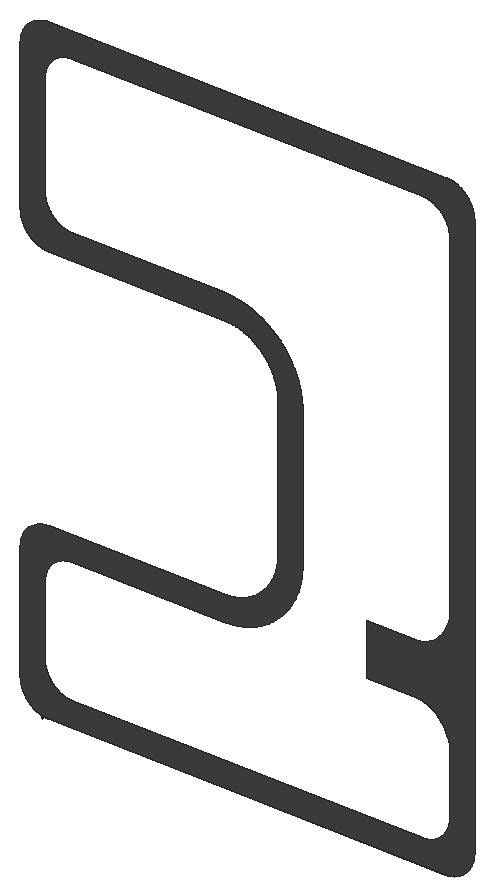
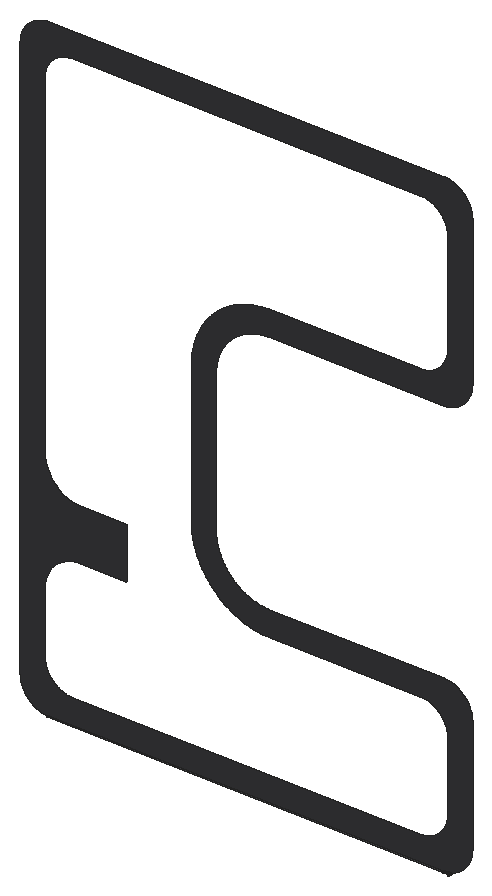
# SketchUp Ruby script. Lengths in inches.
U = 1.inch
M = Sketchup.active_model
def pt(a) = Geom::Point3d.new(a.map { |v| v * U })
def face(e, loops, mat)
  f = e.add_face(loops[0].map { |a| pt(a) })
  loops[1..].each { |l| e.add_face(l.map { |a| pt(a) }).erase! }
  f.material = f.back_material = mat if mat
  f
end
# faces: each face lists its corners as indices into pts; further lists are holes
def faces(e, pts, list, mat = nil) = list.each { |f| face(e, (f[0].is_a?(Array) ? f : [f]).map { |l| l.map { |i| pts[i] } }, mat) }
# xy, xz, yz: faces in a plane at the given z, y or x. An outline is a flat list of corners, or four numbers for a rectangle; further outlines are holes
def ring(l) = l.size == 4 ? [[l[0], l[1]], [l[2], l[1]], [l[2], l[3]], [l[0], l[3]]] : l.each_slice(2).to_a
def flat(e, list, mat, &to3) = list.each { |f| face(e, (f[0].is_a?(Array) ? f : [f]).map { |l| ring(l).map { |u, v| to3.(u, v) } }, mat) }
def xy(e, z, list, mat = nil) = flat(e, list, mat) { |x, y| [x, y, z] }
def xz(e, y, list, mat = nil) = flat(e, list, mat) { |x, z| [x, y, z] }
def yz(e, x, list, mat = nil) = flat(e, list, mat) { |y, z| [x, y, z] }
def lines(e, pts, list) = list.each { |a, b| e.add_line(pt(pts[a]), pt(pts[b])) }
# prism: a flat outline (further loops are holes) pulled along v
def prism(e, loops, v, mat = nil)
  f = face(e, loops, mat); d = Geom::Vector3d.new(v.map { |x| x * U })
  f.pushpull(f.normal.samedirection?(d) ? d.length : -d.length)
end
def box(e, o, s, mat = nil) = prism(e, [[o, [o[0] + s[0], o[1], o[2]], [o[0] + s[0], o[1] + s[1], o[2]], [o[0], o[1] + s[1], o[2]]]], [0, 0, s[2]], mat)
def at(x, y, z, deg = 0) = Geom::Transformation.translation(pt([x, y, z])) * Geom::Transformation.rotation(ORIGIN, Z_AXIS, deg.degrees)
def axes(o, x, y, z) = Geom::Transformation.new([*x, 0, *y, 0, *z, 0, *pt(o).to_a, 1])
def part(name) = M.definitions.add(name)
# library, detail: a bought-in or finely detailed component or shape, given as its bounding box
def library(name, o, s) = part(name).tap { |d| box(d.entities, o, s) }
def detail(e, o, s) = box(e.add_group.entities, o, s)
def put(e, d, t, mat = nil) = e.add_instance(d, t).tap { |i| i.material = mat if mat }
def group(e, t, mat = nil) = e.add_group.tap { |g| g.transformation = t; g.material = mat if mat }.entities
root = M.entities
M.materials.add("1432 AP 8245 TAR ROAD").color = [71, 72, 75]
M.materials.add("Outer Light").color = [251, 217, 152]
xy(root,172.79,[[278.7,95.37,278.85,96.87],[278.85,95.37,279,96.87],[279,95.37,537,96.87],[537,95.37,537.15,96.87],[537.15,95.37,537.3,96.87]],"1432 AP 8245 TAR ROAD")
xy(root,172.79,[[278.7,95.37,278.85,96.87],[278.85,95.37,279,96.87],[279,95.37,537,96.87],[537,95.37,537.15,96.87],[537.15,95.37,537.3,96.87]],"Outer Light")
xy(root,172.8,[[278.4,95.37,278.55,96.87],[537.45,95.37,537.6,96.87]],"1432 AP 8245 TAR ROAD")
xy(root,172.8,[[278.4,95.37,278.55,96.87],[537.45,95.37,537.6,96.87]],"Outer Light")
xz(root,95.37,[[[278.7,172.79,537.3,172.79,537.45,172.8,537.6,172.8,537.75,172.81,537.9,172.8125,538.04,172.82,538.64,172.86,538.79,172.875,538.9375,172.89,539.08,172.91,539.23,172.92,539.68,172.98,539.82,173,539.97,173.03,540.27,173.07,540.41,173.1,540.71,173.16,540.85,173.1875,541,173.22,541.14,173.25,541.29,173.28,541.44,173.32,541.58,173.35,541.73,173.39,542.01,173.47,542.16,173.51,542.44,173.59,542.59,173.63,542.73,173.68,542.87,173.72,543.15,173.82,543.3,173.87,543.4375,173.92,543.58,173.97,543.86,174.07,543.99,174.125,544.13,174.18,544.41,174.3,544.55,174.35,544.68,174.41,544.82,174.48,544.95,174.54,545.09,174.6,545.22,174.66,545.36,174.73,545.49,174.8,545.625,174.86,545.76,174.93,546.28,175.21,546.41,175.29,546.54,175.36,546.67,175.4375,546.8,175.51,546.93,175.59,547.05,175.67,547.31,175.83,547.43,175.91,547.56,175.99,547.68,176.08,547.8,176.16,547.93,176.25,548.05,176.33,548.41,176.6,548.53,176.6875,548.65,176.78,548.76,176.87,548.88,176.96,549,177.06,549.11,177.15,549.23,177.25,549.34,177.34,549.56,177.54,549.68,177.64,550.01,177.94,550.22,178.15,550.33,178.25,550.54,178.46,550.64,178.57,550.75,178.68,550.85,178.79,550.95,178.89,551.05,179,551.15,179.12,551.45,179.45,551.54,179.57,551.64,179.68,551.73,179.8,551.83,179.91,552.1,180.27,552.19,180.38,552.28,180.5,552.46,180.75,552.54,180.87,552.63,180.99,552.71,181.11,552.8,181.24,552.88,181.36,552.96,181.49,553.04,181.61,553.12,181.74,553.2,181.86,553.28,181.99,553.35,182.12,553.43,182.25,553.5,182.38,553.58,182.51,553.86,183.03,553.93,183.17,554,183.3,554.0625,183.43,554.13,183.57,554.19,183.7,554.25,183.84,554.32,183.97,554.38,184.11,554.4375,184.25,554.5,184.38,554.55,184.52,554.67,184.8,554.72,184.9375,554.77,185.08,554.83,185.22,554.875,185.36,554.93,185.5,554.98,185.64,555.02,185.78,555.07,185.92,555.12,186.0625,555.16,186.21,555.2,186.35,555.25,186.49,555.29,186.63,555.33,186.78,555.37,186.92,555.4,187.07,555.44,187.21,555.48,187.36,555.51,187.5,555.54,187.65,555.57,187.79,555.61,187.9375,555.63,188.09,555.66,188.23,555.72,188.53,555.74,188.67,555.77,188.82,555.79,188.97,555.81,189.11,555.89,189.71,555.9,189.86,555.92,190,555.99,191.05,555.99,191.34,556,191.49,556,561.09,555.99,561.24,555.99,561.54,555.98,561.6875,555.97,561.84,555.96,561.99,555.95,562.13,555.92,562.58,555.9,562.73,555.89,562.88,555.87,563.03,555.85,563.17,555.79,563.62,555.77,563.76,555.74,563.91,555.72,564.06,555.69,564.21,555.66,564.35,555.63,564.5,555.61,564.65,555.57,564.79,555.54,564.9375,555.51,565.08,555.48,565.23,555.44,565.37,555.4,565.52,555.37,565.66,555.33,565.81,555.25,566.09,555.2,566.24,555.12,566.52,555.07,566.66,555.02,566.81,554.98,566.95,554.93,567.09,554.875,567.23,554.83,567.37,554.77,567.51,554.67,567.79,554.61,567.92,554.55,568.0625,554.5,568.2,554.4375,568.34,554.38,568.47,554.32,568.61,554.25,568.75,554.19,568.88,554.13,569.02,554.0625,569.15,554,569.28,553.93,569.42,553.79,569.68,553.72,569.8125,553.65,569.95,553.58,570.08,553.5,570.21,553.43,570.34,553.35,570.46,553.28,570.59,553.12,570.85,553.04,570.97,552.96,571.1,552.88,571.22,552.8,571.35,552.71,571.47,552.63,571.59,552.54,571.72,552.46,571.84,552.1,572.32,552.01,572.4375,551.92,572.55,551.83,572.67,551.73,572.79,551.64,572.9,551.54,573.02,551.45,573.13,551.35,573.24,551.25,573.36,551.05,573.58,550.95,573.6875,550.85,573.8,550.75,573.91,550.64,574.01,550.44,574.23,550.33,574.33,550.22,574.4375,550.11,574.54,550.01,574.64,549.9,574.74,549.79,574.85,549.68,574.95,549.56,575.04,549.23,575.34,549.11,575.43,549,575.53,548.76,575.71,548.65,575.8,548.53,575.9,548.29,576.08,548.17,576.16,547.93,576.34,547.8,576.42,547.68,576.51,547.56,576.59,547.43,576.67,547.31,576.75,547.05,576.91,546.93,576.99,546.67,577.15,546.54,577.22,546.41,577.3,545.76,577.65,545.49,577.79,545.36,577.85,545.22,577.92,545.09,577.98,544.95,578.05,544.82,578.11,544.68,578.17,544.55,578.23,544.27,578.35,544.13,578.4,543.99,578.46,543.86,578.51,543.72,578.57,543.58,578.62,543.4375,578.67,543.3,578.72,543.15,578.77,543.01,578.82,542.87,578.86,542.73,578.91,542.59,578.95,542.44,579,542.16,579.08,542.01,579.12,541.73,579.2,541.58,579.23,541.44,579.27,541.14,579.33,541,579.37,540.85,579.4,540.71,579.43,540.56,579.46,540.41,579.48,540.27,579.51,540.12,579.53,539.97,579.56,539.82,579.58,539.68,579.6,539.08,579.68,538.9375,579.69,538.79,579.71,538.04,579.76,537.9,579.77,537.75,579.78,537.6,579.78,537.45,579.79,278.55,579.79,278.4,579.78,278.25,579.78,278.1,579.77,277.96,579.76,277.21,579.71,277.0625,579.69,276.92,579.68,276.32,579.6,276.18,579.58,276.03,579.56,275.88,579.53,275.73,579.51,275.59,579.48,275.44,579.46,275.29,579.43,275.15,579.4,275,579.37,274.86,579.33,274.56,579.27,274.42,579.23,274.27,579.2,273.99,579.12,273.84,579.08,273.56,579,273.41,578.95,273.27,578.91,273.13,578.86,272.99,578.82,272.85,578.77,272.7,578.72,272.5625,578.67,272.42,578.62,272.28,578.57,272.14,578.51,272.01,578.46,271.87,578.4,271.73,578.35,271.45,578.23,271.32,578.17,271.18,578.11,271.05,578.05,270.91,577.98,270.78,577.92,270.64,577.85,270.51,577.79,270.24,577.65,269.59,577.3,269.46,577.22,269.33,577.15,269.07,576.99,268.95,576.91,268.69,576.75,268.57,576.67,268.44,576.59,268.32,576.51,268.2,576.42,268.07,576.34,267.83,576.16,267.71,576.08,267.47,575.9,267.35,575.8,267.24,575.71,267,575.53,266.89,575.43,266.77,575.34,266.44,575.04,266.32,574.95,266.21,574.85,266.1,574.74,265.99,574.64,265.89,574.54,265.78,574.4375,265.67,574.33,265.56,574.23,265.36,574.01,265.25,573.91,265.15,573.8,265.05,573.6875,264.95,573.58,264.75,573.36,264.65,573.24,264.55,573.13,264.46,573.02,264.36,572.9,264.27,572.79,264.17,572.67,264.08,572.55,263.99,572.4375,263.9,572.32,263.54,571.84,263.46,571.72,263.37,571.59,263.29,571.47,263.2,571.35,263.12,571.22,263.04,571.1,262.96,570.97,262.88,570.85,262.72,570.59,262.65,570.46,262.57,570.34,262.5,570.21,262.42,570.08,262.35,569.95,262.28,569.8125,262.21,569.68,262.07,569.42,262,569.28,261.9375,569.15,261.87,569.02,261.81,568.88,261.75,568.75,261.68,568.61,261.62,568.47,261.5625,568.34,261.5,568.2,261.45,568.0625,261.39,567.92,261.33,567.79,261.23,567.51,261.17,567.37,261.125,567.23,261.07,567.09,261.02,566.95,260.98,566.81,260.93,566.66,260.88,566.52,260.8,566.24,260.75,566.09,260.67,565.81,260.63,565.66,260.6,565.52,260.56,565.37,260.52,565.23,260.49,565.08,260.46,564.9375,260.43,564.79,260.39,564.65,260.37,564.5,260.34,564.35,260.31,564.21,260.28,564.06,260.26,563.91,260.23,563.76,260.21,563.62,260.15,563.17,260.13,563.03,260.11,562.88,260.1,562.73,260.08,562.58,260.05,562.13,260.04,561.99,260.03,561.84,260.02,561.6875,260.01,561.54,260.01,561.24,260,561.09,260,464.49,260.01,464.34,260.01,464.05,260.08,463,260.1,462.86,260.11,462.71,260.19,462.11,260.21,461.97,260.23,461.82,260.26,461.67,260.28,461.53,260.34,461.23,260.37,461.09,260.39,460.9375,260.43,460.79,260.46,460.65,260.49,460.5,260.52,460.36,260.56,460.21,260.6,460.07,260.63,459.92,260.67,459.78,260.71,459.63,260.75,459.49,260.8,459.35,260.84,459.21,260.88,459.0625,260.93,458.92,260.98,458.78,261.02,458.64,261.07,458.5,261.125,458.36,261.17,458.22,261.23,458.08,261.28,457.9375,261.33,457.8,261.45,457.52,261.5,457.38,261.5625,457.25,261.62,457.11,261.68,456.97,261.75,456.84,261.81,456.7,261.87,456.57,261.9375,456.43,262,456.3,262.07,456.17,262.14,456.03,262.42,455.51,262.5,455.38,262.57,455.25,262.65,455.12,262.72,454.99,262.8,454.86,262.88,454.74,262.96,454.61,263.04,454.49,263.12,454.36,263.2,454.24,263.29,454.11,263.37,453.99,263.46,453.87,263.54,453.75,263.72,453.5,263.81,453.38,263.9,453.27,264.17,452.91,264.27,452.8,264.36,452.68,264.46,452.57,264.55,452.45,264.85,452.12,264.95,452,265.05,451.89,265.15,451.79,265.25,451.68,265.36,451.57,265.46,451.46,265.67,451.25,265.78,451.15,265.99,450.94,266.32,450.64,266.44,450.54,266.66,450.34,266.77,450.25,266.89,450.15,267,450.06,267.12,449.96,267.24,449.87,267.35,449.78,267.47,449.6875,267.59,449.6,267.95,449.33,268.07,449.25,268.2,449.16,268.32,449.08,268.44,448.99,268.57,448.91,268.69,448.83,268.95,448.67,269.07,448.59,269.2,448.51,269.33,448.4375,269.46,448.36,269.59,448.29,269.72,448.21,270.24,447.93,270.375,447.86,270.51,447.8,270.64,447.73,270.78,447.66,270.91,447.6,271.05,447.54,271.18,447.48,271.32,447.41,271.45,447.35,271.59,447.3,271.87,447.18,272.01,447.125,272.14,447.07,272.42,446.97,272.5625,446.92,272.7,446.87,272.85,446.82,273.13,446.72,273.27,446.68,273.41,446.63,273.56,446.59,273.84,446.51,273.99,446.47,274.27,446.39,274.42,446.35,274.56,446.32,274.71,446.28,274.86,446.25,275,446.22,275.15,446.1875,275.29,446.16,275.59,446.1,275.73,446.07,276.03,446.03,276.18,446,276.32,445.98,276.77,445.92,276.92,445.91,277.0625,445.89,277.21,445.875,277.36,445.86,277.96,445.82,278.1,445.8125,278.25,445.81,278.4,445.8,278.55,445.8,278.7,445.79,393.46,445.79,393.92,445.78,394.375,445.77,394.83,445.74,395.29,445.72,395.75,445.68,396.2,445.65,396.66,445.6,397.11,445.55,397.57,445.49,398.02,445.43,398.48,445.36,398.93,445.29,399.38,445.21,400.28,445.03,400.72,444.93,401.17,444.82,401.62,444.72,402.5,444.48,403.38,444.22,403.82,444.08,405.11,443.63,405.54,443.47,405.97,443.3,406.39,443.13,406.82,442.95,407.24,442.77,407.65,442.58,408.07,442.38,408.89,441.98,409.3,441.77,410.1,441.33,410.9,440.87,411.68,440.39,412.0625,440.15,412.44,439.89,412.82,439.64,413.2,439.375,413.57,439.11,413.94,438.84,414.31,438.56,414.67,438.28,415.03,437.99,415.73,437.41,416.08,437.11,416.76,436.49,417.09,436.18,417.75,435.54,418.39,434.88,418.7,434.55,419.01,434.21,419.3125,433.87,419.61,433.52,419.91,433.17,420.2,432.82,420.49,432.46,420.77,432.1,421.04,431.73,421.32,431.36,421.84,430.62,422.1,430.24,422.35,429.85,422.6,429.47,422.84,429.08,423.08,428.6875,423.3125,428.29,423.54,427.89,423.76,427.49,423.97,427.09,424.19,426.68,424.79,425.45,424.97,425.03,425.16,424.61,425.34,424.1875,425.51,423.76,425.68,423.33,425.84,422.91,425.99,422.48,426.14,422.04,426.29,421.61,426.43,421.17,426.56,420.73,426.6875,420.29,426.81,419.85,426.92,419.41,427.03,418.96,427.14,418.52,427.24,418.07,427.33,417.62,427.57,416.27,427.64,415.8125,427.7,415.36,427.76,414.91,427.81,414.45,427.85,413.99,427.89,413.54,427.93,413.08,427.97,412.17,427.99,411.71,428,411.25,428,320.33,427.99,319.875,427.97,319.42,427.93,318.5,427.89,318.05,427.81,317.13,427.76,316.68,427.7,316.22,427.64,315.77,427.57,315.32,427.49,314.86,427.33,313.96,427.24,313.52,427.14,313.07,427.03,312.62,426.92,312.18,426.81,311.73,426.6875,311.29,426.56,310.85,426.43,310.41,426.29,309.98,426.14,309.54,425.84,308.68,425.68,308.25,425.51,307.82,425.34,307.4,425.16,306.98,424.97,306.56,424.79,306.14,424.59,305.72,424.39,305.3125,424.19,304.9,423.97,304.5,423.76,304.09,423.54,303.69,423.3125,303.29,423.08,302.9,422.84,302.5,422.6,302.12,422.35,301.73,422.1,301.35,421.58,300.59,421.32,300.22,421.04,299.85,420.77,299.49,420.49,299.125,420.2,298.77,419.91,298.41,419.61,298.0625,419.3125,297.71,419.01,297.37,418.7,297.03,418.39,296.7,417.75,296.04,417.09,295.4,416.76,295.09,416.42,294.78,416.08,294.48,415.38,293.88,415.03,293.59,414.67,293.31,414.31,293.02,413.2,292.21,412.44,291.69,412.0625,291.4375,411.68,291.19,410.9,290.71,410.1,290.25,409.7,290.03,409.3,289.82,408.48,289.4,408.07,289.2,407.65,289.01,407.24,288.82,406.82,288.63,406.39,288.46,405.97,288.28,404.68,287.8,404.25,287.65,403.82,287.51,402.94,287.23,402.5,287.11,402.06,286.98,401.62,286.87,401.17,286.76,400.72,286.66,400.28,286.56,399.83,286.46,398.48,286.22,398.02,286.15,397.57,286.09,397.11,286.03,396.66,285.98,396.2,285.9375,395.75,285.9,394.83,285.84,393.92,285.8,393.46,285.8,393,285.79,279,285.79,276.52,285.63,274.08,285.14,271.73,284.35,269.5,283.25,267.43,281.87,265.56,280.23,263.93,278.36,262.55,276.29,261.45,274.0625,260.65,271.71,260.16,269.27,260,266.79,260,191.49,260.01,191.34,260.01,191.05,260.08,190,260.1,189.86,260.11,189.71,260.19,189.11,260.21,188.97,260.23,188.82,260.26,188.67,260.28,188.53,260.34,188.23,260.37,188.09,260.39,187.9375,260.43,187.79,260.46,187.65,260.49,187.5,260.52,187.36,260.56,187.21,260.6,187.07,260.63,186.92,260.67,186.78,260.71,186.63,260.75,186.49,260.8,186.35,260.84,186.21,260.88,186.0625,260.93,185.92,260.98,185.78,261.02,185.64,261.07,185.5,261.125,185.36,261.17,185.22,261.23,185.08,261.28,184.9375,261.33,184.8,261.45,184.52,261.5,184.38,261.5625,184.25,261.62,184.11,261.68,183.97,261.75,183.84,261.81,183.7,261.87,183.57,261.9375,183.43,262,183.3,262.07,183.17,262.14,183.03,262.42,182.51,262.5,182.38,262.57,182.25,262.65,182.12,262.72,181.99,262.8,181.86,262.88,181.74,262.96,181.61,263.04,181.49,263.12,181.36,263.2,181.24,263.29,181.11,263.37,180.99,263.46,180.87,263.54,180.75,263.72,180.5,263.81,180.38,263.9,180.27,264.17,179.91,264.27,179.8,264.36,179.68,264.46,179.57,264.55,179.45,264.85,179.12,264.95,179,265.05,178.89,265.15,178.79,265.25,178.68,265.36,178.57,265.46,178.46,265.67,178.25,265.78,178.15,265.99,177.94,266.32,177.64,266.44,177.54,266.66,177.34,266.77,177.25,266.89,177.15,267,177.06,267.12,176.96,267.24,176.87,267.35,176.78,267.47,176.6875,267.59,176.6,267.95,176.33,268.07,176.25,268.2,176.16,268.32,176.08,268.44,175.99,268.57,175.91,268.69,175.83,268.95,175.67,269.07,175.59,269.2,175.51,269.33,175.4375,269.46,175.36,269.59,175.29,269.72,175.21,270.24,174.93,270.375,174.86,270.51,174.8,270.64,174.73,270.78,174.66,270.91,174.6,271.05,174.54,271.18,174.48,271.32,174.41,271.45,174.35,271.59,174.3,271.87,174.18,272.01,174.125,272.14,174.07,272.42,173.97,272.5625,173.92,272.7,173.87,272.85,173.82,273.13,173.72,273.27,173.68,273.41,173.63,273.56,173.59,273.84,173.51,273.99,173.47,274.27,173.39,274.42,173.35,274.56,173.32,274.71,173.28,274.86,173.25,275,173.22,275.15,173.1875,275.29,173.16,275.59,173.1,275.73,173.07,276.03,173.03,276.18,173,276.32,172.98,276.77,172.92,276.92,172.91,277.0625,172.89,277.21,172.875,277.36,172.86,277.96,172.82,278.1,172.8125,278.25,172.81,278.4,172.8,278.55,172.8],[293.76,188.79,293.53,188.8,293.29,188.81,293.06,188.82,292.82,188.83,292.59,188.85,292.35,188.87,292.12,188.89,291.88,188.92,291.42,188.98,291.18,189.01,290.72,189.09,289.8,189.29,289.11,189.47,288.89,189.53,288.66,189.6,288.4375,189.67,288.21,189.75,287.99,189.82,287.77,189.9,287.55,189.99,287.33,190.07,286.89,190.25,286.68,190.35,286.46,190.45,285.83,190.75,285.41,190.97,285.2,191.09,285,191.2,284.6,191.44,284.39,191.57,284.2,191.7,283.8,191.96,283.61,192.09,283.04,192.51,282.86,192.66,282.67,192.8,282.31,193.1,282.13,193.26,281.96,193.42,281.78,193.57,281.61,193.74,281.44,193.9,281.27,194.0625,281.11,194.23,280.94,194.4,280.78,194.57,280.625,194.75,280.47,194.92,280.3125,195.1,280.16,195.28,280.01,195.46,279.86,195.65,279.72,195.83,279.58,196.02,279.4375,196.21,279.3,196.4,279.17,196.6,279.03,196.79,278.9,196.99,278.78,197.1875,278.65,197.39,278.41,197.79,278.3,198,278.18,198.2,277.96,198.62,277.86,198.83,277.75,199.04,277.65,199.26,277.56,199.47,277.46,199.6875,277.37,199.9,277.28,200.12,277.2,200.34,277.11,200.5625,277.03,200.78,276.96,201.01,276.88,201.23,276.81,201.45,276.74,201.68,276.68,201.91,276.61,202.13,276.55,202.36,276.5,202.59,276.44,202.82,276.39,203.05,276.35,203.28,276.3,203.51,276.26,203.74,276.22,203.98,276.1875,204.21,276.15,204.44,276.125,204.68,276.1,204.91,276.08,205.15,276.04,205.61,276.02,205.85,276.01,206.09,276.01,206.32,276,206.56,276,252.19,276.01,252.4,276.04,253,276.06,253.2,276.07,253.4,276.11,253.8,276.14,254,276.16,254.2,276.25,254.8,276.29,255,276.32,255.2,276.36,255.39,276.41,255.59,276.45,255.79,276.49,255.98,276.54,256.18,276.59,256.375,276.65,256.57,276.7,256.76,276.76,256.96,276.82,257.15,276.875,257.34,277,257.72,277.21,258.29,277.29,258.48,277.36,258.66,277.44,258.85,277.52,259.03,277.6,259.22,277.6875,259.4,277.77,259.58,278.04,260.12,278.14,260.3,278.23,260.48,278.33,260.65,278.43,260.83,278.53,261,278.64,261.17,278.74,261.35,278.85,261.52,278.96,261.68,279.07,261.85,279.1875,262.02,279.3,262.18,279.42,262.35,279.78,262.83,279.91,262.99,280.03,263.15,280.16,263.3,280.29,263.46,280.55,263.76,280.6875,263.91,280.83,264.06,280.96,264.2,281.1,264.35,281.24,264.49,281.39,264.63,281.53,264.77,281.83,265.05,282,265.16,282.16,265.3125,282.33,265.46,282.49,265.61,282.67,265.76,282.84,265.9,283.01,266.03,283.19,266.17,283.37,266.3,283.56,266.43,283.74,266.55,284.12,266.79,284.27,266.9375,284.45,267.05,284.81,267.27,285.17,267.48,285.36,267.58,285.54,267.68,285.73,267.78,285.91,267.87,286.1,267.97,286.48,268.15,286.67,268.23,286.86,268.32,287.06,268.4,287.44,268.56,287.84,268.7,288.03,268.77,288.43,268.91,289.23,269.15,289.4375,269.2,289.64,269.26,289.84,269.31,290.05,269.35,290.25,269.4,290.46,269.44,290.66,269.48,290.87,269.52,291.08,269.55,291.28,269.59,291.49,269.62,291.7,269.64,291.91,269.67,292.12,269.69,292.32,269.71,292.74,269.75,293.58,269.79,393,269.79,394.34,269.81,395,269.83,395.67,269.86,396.34,269.9,397,269.95,397.67,270.01,398.33,270.07,398.99,270.15,399.66,270.23,400.32,270.32,400.98,270.42,401.64,270.53,402.29,270.65,402.95,270.77,403.6,270.91,404.26,271.05,404.91,271.2,405.55,271.36,406.2,271.53,407.48,271.89,408.125,272.09,408.76,272.29,409.39,272.5,410.65,272.94,411.28,273.18,411.9,273.42,412.52,273.67,413.13,273.93,413.74,274.2,414.96,274.76,415.56,275.05,416.15,275.35,416.75,275.66,417.34,275.97,417.92,276.29,419.08,276.96,419.65,277.31,420.21,277.66,420.78,278.02,421.33,278.39,421.89,278.76,422.43,279.14,422.98,279.53,423.51,279.93,424.05,280.33,424.57,280.74,425.1,281.16,425.61,281.58,426.12,282.01,426.625,282.45,427.125,282.89,427.62,283.34,428.11,283.8,428.59,284.26,429.0625,284.73,429.53,285.2,429.99,285.6875,430.45,286.17,430.9,286.67,431.78,287.67,432.21,288.18,433.05,289.22,433.46,289.75,433.86,290.28,434.26,290.82,434.65,291.36,435.03,291.91,435.4,292.46,435.77,293.02,436.13,293.58,436.48,294.14,436.83,294.72,437.17,295.29,437.5,295.87,437.82,296.46,438.44,297.64,438.74,298.24,439.32,299.44,439.86,300.66,440.12,301.28,440.37,301.89,440.61,302.52,440.85,303.14,441.29,304.4,441.5,305.03,441.71,305.67,442.09,306.95,442.26,307.59,442.43,308.24,442.59,308.89,442.74,309.54,442.89,310.1875,443.02,310.84,443.15,311.5,443.26,312.16,443.37,312.8125,443.47,313.47,443.5625,314.14,443.65,314.8,443.72,315.46,443.79,316.125,443.84,316.79,443.89,317.46,443.93,318.12,443.96,318.79,443.98,319.46,444,320.125,444,411.46,443.98,412.13,443.96,412.79,443.93,413.46,443.89,414.13,443.84,414.79,443.79,415.46,443.65,416.79,443.5625,417.45,443.47,418.11,443.37,418.77,443.15,420.09,443.02,420.74,442.89,421.4,442.59,422.7,442.43,423.35,442.26,423.99,442.09,424.64,441.71,425.92,441.5,426.55,441.29,427.19,441.07,427.82,440.85,428.44,440.61,429.07,440.37,429.69,440.12,430.31,439.86,430.92,439.59,431.54,439.32,432.14,439.03,432.75,438.74,433.35,438.44,433.95,437.82,435.13,437.5,435.71,437.17,436.29,436.83,436.87,436.48,437.4375,436.13,438.01,435.77,438.57,435.03,439.68,434.65,440.23,434.26,440.77,433.86,441.31,433.46,441.84,433.05,442.37,432.63,442.89,432.21,443.4,431.78,443.91,431.34,444.42,430.9,444.92,430.45,445.41,429.99,445.9,429.53,446.38,429.0625,446.85,428.59,447.32,428.11,447.79,427.62,448.24,427.125,448.69,426.625,449.14,426.12,449.57,425.1,450.43,424.57,450.84,424.05,451.25,423.51,451.66,422.98,452.05,422.43,452.44,421.89,452.82,421.33,453.2,420.78,453.5625,420.21,453.92,419.65,454.28,419.08,454.62,418.5,454.96,417.92,455.29,417.34,455.61,416.75,455.93,416.15,456.23,415.56,456.53,414.96,456.82,414.35,457.11,413.13,457.65,412.52,457.91,411.9,458.16,411.28,458.4,410.65,458.64,410.02,458.87,409.39,459.09,408.76,459.3,408.125,459.5,407.48,459.69,406.84,459.88,406.2,460.05,405.55,460.22,404.91,460.38,404.26,460.53,403.6,460.68,402.95,460.8125,402.29,460.9375,401.64,461.06,399.66,461.36,398.99,461.4375,398.33,461.51,397.67,461.58,397,461.63,396.34,461.68,395.67,461.72,395,461.75,394.34,461.77,393.67,461.79,293.76,461.79,293.53,461.8,293.29,461.81,293.06,461.82,292.82,461.83,292.59,461.85,292.35,461.87,292.12,461.89,291.88,461.92,291.42,461.98,291.18,462.01,290.72,462.09,289.8,462.29,289.11,462.47,288.89,462.53,288.66,462.6,288.4375,462.67,288.21,462.75,287.99,462.82,287.77,462.9,287.55,462.99,287.33,463.07,286.89,463.25,286.68,463.35,286.46,463.45,285.83,463.75,285.41,463.97,285.2,464.09,285,464.2,284.6,464.44,284.39,464.57,284.2,464.7,283.8,464.96,283.61,465.09,283.04,465.51,282.86,465.66,282.67,465.8,282.31,466.1,282.13,466.26,281.96,466.42,281.78,466.57,281.61,466.74,281.44,466.9,281.27,467.0625,281.11,467.23,280.94,467.4,280.78,467.57,280.625,467.75,280.47,467.92,280.3125,468.1,280.16,468.28,280.01,468.46,279.86,468.65,279.72,468.83,279.58,469.02,279.4375,469.21,279.3,469.4,279.17,469.6,279.03,469.79,278.9,469.99,278.78,470.1875,278.65,470.39,278.41,470.79,278.3,471,278.18,471.2,277.96,471.62,277.86,471.83,277.75,472.04,277.65,472.26,277.56,472.47,277.46,472.6875,277.37,472.9,277.28,473.12,277.2,473.34,277.11,473.5625,277.03,473.78,276.96,474.01,276.88,474.23,276.81,474.45,276.74,474.68,276.68,474.91,276.61,475.13,276.55,475.36,276.5,475.59,276.44,475.82,276.39,476.05,276.35,476.28,276.3,476.51,276.26,476.74,276.22,476.98,276.1875,477.21,276.15,477.44,276.125,477.68,276.1,477.91,276.08,478.15,276.04,478.61,276.02,478.85,276.01,479.09,276.01,479.32,276,479.56,276,546.03,276.01,546.26,276.01,546.5,276.02,546.73,276.04,546.97,276.06,547.2,276.08,547.4375,276.1,547.67,276.125,547.91,276.15,548.14,276.1875,548.375,276.22,548.61,276.3,549.07,276.35,549.3,276.39,549.53,276.44,549.76,276.5,549.99,276.55,550.22,276.61,550.45,276.68,550.68,276.74,550.9,276.81,551.13,276.88,551.35,276.96,551.58,277.03,551.8,277.11,552.02,277.2,552.24,277.28,552.46,277.46,552.9,277.56,553.11,277.65,553.33,277.75,553.54,277.86,553.75,277.96,553.96,278.18,554.38,278.3,554.59,278.41,554.79,278.53,555,278.65,555.2,278.78,555.4,278.9,555.6,279.03,555.79,279.17,555.99,279.3,556.18,279.4375,556.37,279.58,556.5625,279.86,556.9375,280.01,557.12,280.16,557.3,280.3125,557.48,280.47,557.66,280.625,557.84,280.78,558.01,280.94,558.18,281.11,558.35,281.27,558.52,281.44,558.69,281.78,559.01,281.96,559.17,282.13,559.33,282.67,559.78,282.86,559.93,283.04,560.07,283.61,560.49,283.8,560.625,284,560.76,284.2,560.89,284.39,561.02,284.6,561.14,285.2,561.5,285.83,561.83,286.04,561.9375,286.25,562.04,286.46,562.14,286.68,562.24,286.89,562.33,287.55,562.6,288.21,562.84,288.4375,562.91,288.66,562.98,288.89,563.05,289.11,563.12,289.57,563.24,289.8,563.29,290.03,563.35,290.49,563.45,291.18,563.57,291.42,563.61,291.88,563.67,292.12,563.69,292.35,563.72,292.59,563.74,292.82,563.75,293.06,563.77,293.29,563.78,293.53,563.79,522.4,563.79,522.61,563.78,523.41,563.74,523.81,563.7,524.02,563.68,524.22,563.66,525.02,563.54,525.21,563.5,525.41,563.47,525.61,563.43,525.81,563.38,526.01,563.34,526.2,563.29,526.4,563.25,526.59,563.2,526.79,563.14,526.98,563.09,527.18,563.03,527.37,562.97,527.5625,562.91,527.75,562.85,527.95,562.78,528.14,562.71,528.32,562.64,528.7,562.5,528.89,562.42,529.07,562.34,529.26,562.26,529.44,562.18,529.63,562.1,530.35,561.74,530.53,561.64,530.71,561.55,530.88,561.45,531.06,561.35,531.23,561.24,531.4,561.14,531.58,561.03,531.75,560.92,531.92,560.8125,532.08,560.7,532.25,560.59,532.42,560.47,532.9,560.11,533.0625,559.99,533.22,559.87,533.54,559.61,533.84,559.35,533.99,559.21,534.14,559.08,534.29,558.94,534.4375,558.8,534.58,558.66,534.73,558.52,535.01,558.23,535.15,558.08,535.29,557.9375,535.42,557.79,535.56,557.63,535.6875,557.48,535.82,557.33,535.95,557.17,536.07,557.01,536.2,556.86,536.32,556.7,536.44,556.53,536.5625,556.37,536.68,556.21,536.8,556.04,537.02,555.71,537.35,555.2,537.45,555.02,537.55,554.85,537.66,554.68,537.75,554.5,537.95,554.14,538.22,553.6,538.3,553.42,538.39,553.24,538.47,553.05,538.55,552.87,538.71,552.49,538.78,552.31,539.06,551.55,539.12,551.35,539.3,550.78,539.35,550.58,539.4,550.39,539.5,549.99,539.55,549.8,539.67,549.2,539.71,549.01,539.75,548.81,539.84,548.21,539.86,548.01,539.89,547.81,539.93,547.41,539.94,547.2,539.96,547,540,546.2,540,326.79,539.79,323.66,539.18,320.58,538.17,317.61,536.78,314.79,535.04,312.18,532.97,309.82,530.61,307.75,528,306.01,525.18,304.62,522.21,303.61,519.13,303,516,302.79,486,302.79,486,269.79,516,269.79,519.13,269.59,522.21,268.97,525.18,267.97,528,266.58,530.61,264.83,532.97,262.76,535.04,260.4,536.78,257.79,538.17,254.98,539.18,252,539.79,248.92,540,245.79,540,206.39,539.99,206.1875,539.98,205.98,539.96,205.58,539.94,205.38,539.93,205.18,539.89,204.78,539.86,204.58,539.84,204.375,539.81,204.18,539.75,203.78,539.59,202.98,539.55,202.79,539.45,202.39,539.4,202.2,539.35,202,539.3,201.81,539.24,201.62,539.18,201.42,539.06,201.04,538.71,200.09,538.63,199.9,538.55,199.72,538.47,199.53,538.39,199.35,538.3,199.16,538.22,198.98,537.95,198.44,537.85,198.26,537.75,198.09,537.66,197.91,537.55,197.73,537.35,197.39,537.13,197.05,537.02,196.875,536.91,196.71,536.8,196.54,536.68,196.375,536.5625,196.21,536.44,196.05,536.2,195.73,536.07,195.57,535.95,195.41,535.82,195.26,535.6875,195.1,535.56,194.95,535.42,194.8,535.29,194.65,535.01,194.35,534.87,194.21,534.73,194.0625,534.58,193.92,534.4375,193.78,534.29,193.64,534.14,193.51,533.99,193.37,533.84,193.24,533.69,193.1,533.54,192.97,533.38,192.85,533.22,192.72,533.0625,192.59,532.9,192.47,532.42,192.11,532.25,192,532.08,191.88,531.92,191.77,531.58,191.55,531.4,191.44,531.06,191.24,530.88,191.14,530.71,191.04,530.53,190.94,530.35,190.85,530.17,190.75,529.81,190.57,529.63,190.49,529.44,190.4,529.26,190.32,529.07,190.24,528.89,190.16,528.7,190.09,528.51,190.01,528.32,189.94,528.14,189.87,527.95,189.8,527.75,189.74,527.5625,189.67,527.37,189.61,527.18,189.55,526.98,189.5,526.79,189.44,526.59,189.39,526.4,189.34,526.2,189.29,526.01,189.24,525.21,189.08,525.02,189.05,524.82,189.01,524.42,188.95,524.02,188.91,523.81,188.88,523.61,188.86,523.41,188.85,523.21,188.83,522.61,188.8,522.4,188.8,522.2,188.79]]],"1432 AP 8245 TAR ROAD")
p = [[274.21,95.37,171.86],[274.37,95.37,171.82],[274.37,96.87,171.82],[274.21,96.87,171.86],[274.21,96.87,171.86],[274.37,96.87,171.82],
  [274.37,95.37,171.82],[274.21,95.37,171.86],[274.53,95.37,171.79],[274.53,96.87,171.79],[274.53,96.87,171.79],[274.53,95.37,171.79],
  [274.69,95.37,171.75],[274.69,96.87,171.75],[274.69,96.87,171.75],[274.69,95.37,171.75],[273.75,95.37,171.98],[273.9,95.37,171.9375],
  [273.9,96.87,171.9375],[273.75,96.87,171.98],[273.75,96.87,171.98],[273.9,96.87,171.9375],[273.9,95.37,171.9375],[273.75,95.37,171.98],
  [274.06,95.37,171.9],[274.06,96.87,171.9],[274.06,96.87,171.9],[274.06,95.37,171.9],[277.66,95.37,172.84],[277.51,95.37,172.85],
  [277.51,96.87,172.85],[277.66,96.87,172.84],[277.66,96.87,172.84],[277.51,96.87,172.85],[277.51,95.37,172.85],[277.66,95.37,172.84],
  [277.81,95.37,172.83],[277.81,96.87,172.83],[277.81,96.87,172.83],[277.81,95.37,172.83],[277.96,95.37,172.82],[277.96,96.87,172.82],
  [277.96,96.87,172.82],[277.96,95.37,172.82],[278.1,95.37,172.8125],[278.1,96.87,172.8125],[278.1,96.87,172.8125],[278.1,95.37,172.8125],
  [278.25,95.37,172.81],[278.25,96.87,172.81],[278.25,96.87,172.81],[278.25,95.37,172.81],[278.4,95.37,172.8],[278.4,96.87,172.8],
  [278.4,96.87,172.8],[278.4,95.37,172.8],[278.7,95.37,172.79],[278.55,95.37,172.8],[278.55,96.87,172.8],[278.7,96.87,172.79],
  [278.7,96.87,172.79],[278.55,96.87,172.8],[278.55,95.37,172.8],[278.7,95.37,172.79],[537.45,95.37,172.8],[537.3,95.37,172.79],
  [537.3,96.87,172.79],[537.45,96.87,172.8],[537.45,96.87,172.8],[537.3,96.87,172.79],[537.3,95.37,172.79],[537.45,95.37,172.8],
  [276.62,95.37,172.94],[276.47,95.37,172.96],[276.47,96.87,172.96],[276.62,96.87,172.94],[276.62,96.87,172.94],[276.47,96.87,172.96],
  [276.47,95.37,172.96],[276.62,95.37,172.94],[276.77,95.37,172.92],[276.77,96.87,172.92],[276.77,96.87,172.92],[276.77,95.37,172.92],
  [276.92,95.37,172.91],[276.92,96.87,172.91],[276.92,96.87,172.91],[276.92,95.37,172.91],[277.0625,95.37,172.89],[277.0625,96.87,172.89],
  [277.0625,96.87,172.89],[277.0625,95.37,172.89],[277.21,95.37,172.875],[277.21,96.87,172.875],[277.21,96.87,172.875],[277.21,95.37,172.875],
  [277.36,95.37,172.86],[277.36,96.87,172.86],[277.36,96.87,172.86],[277.36,95.37,172.86],[275.88,95.37,173.05],[275.73,95.37,173.07],
  [275.73,96.87,173.07],[275.88,96.87,173.05],[275.88,96.87,173.05],[275.73,96.87,173.07],[275.73,95.37,173.07],[275.88,95.37,173.05],
  [276.03,95.37,173.03],[276.03,96.87,173.03],[276.03,96.87,173.03],[276.03,95.37,173.03],[276.18,95.37,173],[276.18,96.87,173],
  [276.18,96.87,173],[276.18,95.37,173],[276.32,95.37,172.98],[276.32,96.87,172.98],[276.32,96.87,172.98],[276.32,95.37,172.98],
  [275.44,95.37,173.13],[275.29,95.37,173.16],[275.29,96.87,173.16],[275.44,96.87,173.13],[275.44,96.87,173.13],[275.29,96.87,173.16],
  [275.29,95.37,173.16],[275.44,95.37,173.13],[275.59,95.37,173.1],[275.59,96.87,173.1],[275.59,96.87,173.1],[275.59,95.37,173.1],
  [274.86,95.37,173.25],[274.71,95.37,173.28],[274.71,96.87,173.28],[274.86,96.87,173.25],[274.86,96.87,173.25],[274.71,96.87,173.28],
  [274.71,95.37,173.28],[274.86,95.37,173.25],[275,95.37,173.22],[275,96.87,173.22],[275,96.87,173.22],[275,95.37,173.22],
  [275.15,95.37,173.1875],[275.15,96.87,173.1875],[275.15,96.87,173.1875],[275.15,95.37,173.1875],[274.56,95.37,173.32],[274.42,95.37,173.35],
  [274.42,96.87,173.35],[274.56,96.87,173.32],[274.56,96.87,173.32],[274.42,96.87,173.35],[274.42,95.37,173.35],[274.56,95.37,173.32],
  [274.13,95.37,173.43],[273.99,95.37,173.47],[273.99,96.87,173.47],[274.13,96.87,173.43],[274.13,96.87,173.43],[273.99,96.87,173.47],
  [273.99,95.37,173.47],[274.13,95.37,173.43],[274.27,95.37,173.39],[274.27,96.87,173.39],[274.27,96.87,173.39],[274.27,95.37,173.39],
  [273.84,95.37,173.51],[273.84,96.87,173.51],[273.84,96.87,173.51],[273.84,95.37,173.51]]
faces(root,p,[[0,1,2,3],[1,8,9,2],[8,12,13,9],[16,17,18,19],[17,24,25,18],[24,0,3,25],[28,29,30,31],[36,28,31,37],
  [40,36,37,41],[44,40,41,45],[48,44,45,49],[52,48,49,53],[56,57,58,59],[64,65,66,67],[72,73,74,75],[80,72,75,81],
  [84,80,81,85],[88,84,85,89],[92,88,89,93],[96,92,93,97],[29,96,97,30],[100,101,102,103],[108,100,103,109],[112,108,109,113],
  [116,112,113,117],[73,116,117,74],[120,121,122,123],[128,120,123,129],[101,128,129,102],[132,133,134,135],[140,132,135,141],[144,140,141,145],
  [121,144,145,122],[148,149,150,151],[133,148,151,134],[156,157,158,159],[164,156,159,165],[149,164,165,150],[157,168,169,158]],"1432 AP 8245 TAR ROAD")
faces(root,p,[[4,5,6,7],[5,10,11,6],[10,14,15,11],[20,21,22,23],[21,26,27,22],[26,4,7,27],[32,33,34,35],[38,32,35,39],
  [42,38,39,43],[46,42,43,47],[50,46,47,51],[54,50,51,55],[60,61,62,63],[68,69,70,71],[76,77,78,79],[82,76,79,83],
  [86,82,83,87],[90,86,87,91],[94,90,91,95],[98,94,95,99],[33,98,99,34],[104,105,106,107],[110,104,107,111],[114,110,111,115],
  [118,114,115,119],[77,118,119,78],[124,125,126,127],[130,124,127,131],[105,130,131,106],[136,137,138,139],[142,136,139,143],[146,142,143,147],
  [125,146,147,126],[152,153,154,155],[137,152,155,138],[160,161,162,163],[166,160,163,167],[153,166,167,154],[161,170,171,162]],"Outer Light")
